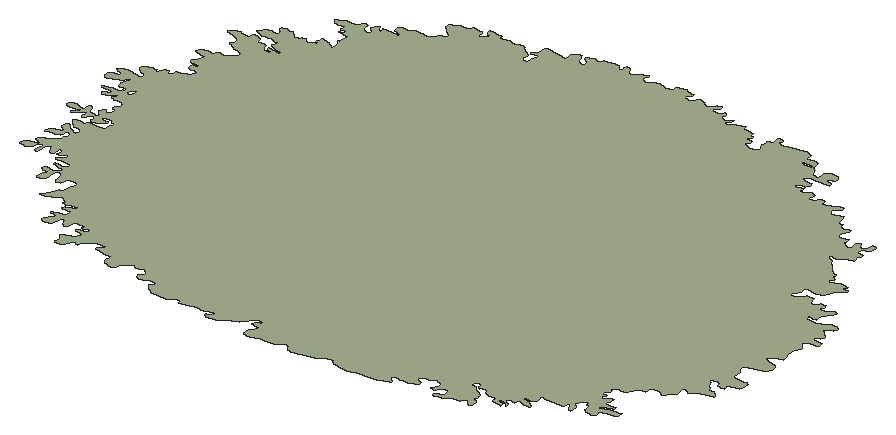
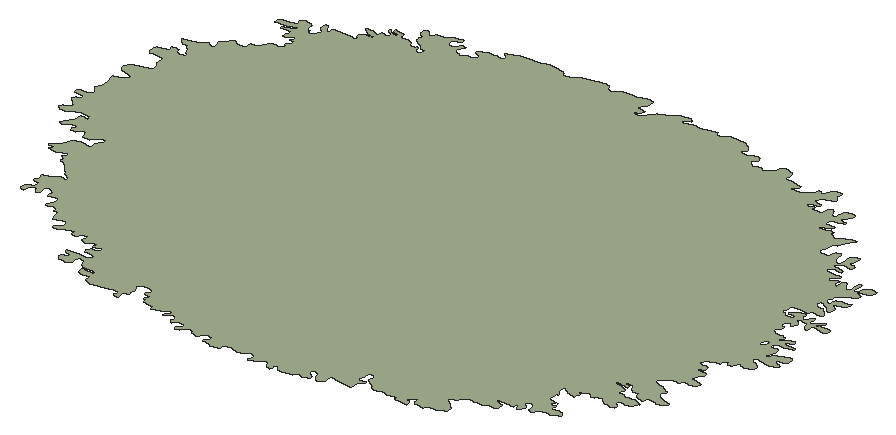
# SketchUp Ruby script. Lengths in inches.
U = 1.inch
M = Sketchup.active_model
def pt(a) = Geom::Point3d.new(a.map { |v| v * U })
def face(e, loops, mat)
  f = e.add_face(loops[0].map { |a| pt(a) })
  loops[1..].each { |l| e.add_face(l.map { |a| pt(a) }).erase! }
  f.material = f.back_material = mat if mat
  f
end
# faces: each face lists its corners as indices into pts; further lists are holes
def faces(e, pts, list, mat = nil) = list.each { |f| face(e, (f[0].is_a?(Array) ? f : [f]).map { |l| l.map { |i| pts[i] } }, mat) }
# xy, xz, yz: faces in a plane at the given z, y or x. An outline is a flat list of corners, or four numbers for a rectangle; further outlines are holes
def ring(l) = l.size == 4 ? [[l[0], l[1]], [l[2], l[1]], [l[2], l[3]], [l[0], l[3]]] : l.each_slice(2).to_a
def flat(e, list, mat, &to3) = list.each { |f| face(e, (f[0].is_a?(Array) ? f : [f]).map { |l| ring(l).map { |u, v| to3.(u, v) } }, mat) }
def xy(e, z, list, mat = nil) = flat(e, list, mat) { |x, y| [x, y, z] }
def xz(e, y, list, mat = nil) = flat(e, list, mat) { |x, z| [x, y, z] }
def yz(e, x, list, mat = nil) = flat(e, list, mat) { |y, z| [x, y, z] }
def lines(e, pts, list) = list.each { |a, b| e.add_line(pt(pts[a]), pt(pts[b])) }
# prism: a flat outline (further loops are holes) pulled along v
def prism(e, loops, v, mat = nil)
  f = face(e, loops, mat); d = Geom::Vector3d.new(v.map { |x| x * U })
  f.pushpull(f.normal.samedirection?(d) ? d.length : -d.length)
end
def box(e, o, s, mat = nil) = prism(e, [[o, [o[0] + s[0], o[1], o[2]], [o[0] + s[0], o[1] + s[1], o[2]], [o[0], o[1] + s[1], o[2]]]], [0, 0, s[2]], mat)
def at(x, y, z, deg = 0) = Geom::Transformation.translation(pt([x, y, z])) * Geom::Transformation.rotation(ORIGIN, Z_AXIS, deg.degrees)
def axes(o, x, y, z) = Geom::Transformation.new([*x, 0, *y, 0, *z, 0, *pt(o).to_a, 1])
def part(name) = M.definitions.add(name)
# library, detail: a bought-in or finely detailed component or shape, given as its bounding box
def library(name, o, s) = part(name).tap { |d| box(d.entities, o, s) }
def detail(e, o, s) = box(e.add_group.entities, o, s)
def put(e, d, t, mat = nil) = e.add_instance(d, t).tap { |i| i.material = mat if mat }
def group(e, t, mat = nil) = e.add_group.tap { |g| g.transformation = t; g.material = mat if mat }.entities
root = M.entities
M.materials.add("Boxwoodplan").color = [166, 177, 144]
xy(root,9.058,[[[199.667,67.129,199.556,67.133,199.461,67.159,199.405,67.215,199.403,67.317,199.429,67.382,199.493,67.445,199.542,67.509,199.6,67.606,199.414,67.635,199.324,67.644,199.344,67.732,199.43,67.79,199.461,67.8,199.456,67.846,199.367,67.877,199.251,67.837,199.154,67.706,199.011,67.551,198.85,67.464,198.745,67.441,198.684,67.416,198.668,67.373,198.524,67.281,198.33,67.251,198.241,67.26,198.161,67.306,198.161,67.328,198.206,67.359,198.297,67.437,198.365,67.483,198.276,67.498,198.163,67.48,198.043,67.436,197.947,67.445,197.85,67.454,197.753,67.447,197.626,67.403,197.426,67.356,197.337,67.349,197.299,67.443,197.291,67.465,197.224,67.473,197.135,67.454,196.966,67.336,196.766,67.328,196.536,67.353,196.369,67.446,196.228,67.61,196.411,67.702,196.311,67.756,196.175,67.772,196.049,67.749,195.977,67.697,195.896,67.672,195.78,67.738,195.738,67.806,195.826,67.847,195.852,67.907,195.857,67.957,195.816,68.009,195.744,68.085,195.658,68.117,195.571,68.064,195.505,68.038,195.449,68.08,195.432,68.103,195.408,68.121,195.379,68.111,195.299,68.058,195.228,68.01,195.152,67.923,195.14,67.79,195.069,67.749,195.019,67.723,194.959,67.725,194.86,67.746,194.773,67.793,194.729,67.861,194.721,67.951,194.73,68.018,194.743,68.04,194.724,68.08,194.51,68.1,194.578,68.135,194.552,68.136,194.459,68.13,194.289,68.146,194.212,68.173,194.195,68.206,194.21,68.224,194.335,68.314,194.333,68.371,194.248,68.393,194.089,68.39,193.958,68.319,193.861,68.233,193.786,68.199,193.739,68.172,193.738,68.154,193.774,68.101,193.758,68.046,193.688,68.081,193.624,68.121,193.563,68.072,193.541,68.017,193.509,67.904,193.462,67.855,193.389,67.822,193.298,67.816,193.228,67.841,193.209,67.874,193.216,67.892,193.237,67.932,193.259,67.991,193.228,68.048,193.127,68.149,193.241,68.229,193.302,68.269,193.382,68.285,193.449,68.315,193.504,68.37,193.589,68.476,193.517,68.503,193.4375,68.511,193.305,68.53,193.267,68.565,193.274,68.584,193.349,68.62,193.511,68.657,193.553,68.709,193.548,68.748,193.522,68.764,193.372,68.711,193.326,68.732,193.327,68.752,193.35,68.814,193.189,68.825,193.108,68.833,193.054,68.826,193.047,68.806,193.031,68.71,193.016,68.642,192.974,68.591,192.927,68.578,192.908,68.594,192.849,68.639,192.804,68.757,192.765,68.783,192.738,68.784,192.684,68.777,192.677,68.757,192.675,68.641,192.621,68.523,192.56,68.449,192.48,68.419,192.401,68.422,192.355,68.448,192.322,68.506,192.322,68.564,192.376,68.677,192.49,68.784,192.51,68.803,192.497,68.823,192.47,68.829,192.39,68.847,192.309,68.86,192.282,68.875,192.289,68.895,192.309,68.914,192.458,68.982,192.62,69.005,192.662,69.108,192.635,69.169,192.588,69.191,192.561,69.187,192.398,69.168,192.357,69.2,192.364,69.22,192.391,69.279,192.549,69.334,192.721,69.403,192.769,69.442,192.756,69.463,192.659,69.436,192.488,69.417,192.344,69.372,192.255,69.386,192.228,69.392,192.234,69.412,192.255,69.426,192.31,69.47,192.282,69.507,192.255,69.503,192.172,69.511,192.117,69.56,192.103,69.601,192.076,69.597,191.993,69.575,191.836,69.489,191.687,69.413,191.613,69.38,191.558,69.392,191.571,69.412,191.59,69.452,191.617,69.469,191.641,69.55,191.691,69.65,191.723,69.759,191.774,69.812,191.847,69.852,191.891,69.972,191.913,70.112,191.933,70.227,191.929,70.285,191.884,70.321,191.803,70.335,191.717,70.335,191.643,70.31,191.633,70.245,191.634,70.184,191.601,70.124,191.513,70.087,191.456,70.096,191.418,70.155,191.407,70.216,191.381,70.337,191.376,70.4,191.335,70.453,191.308,70.475,191.27,70.491,191.211,70.479,191.177,70.46,191.175,70.428,191.167,70.366,191.17,70.229,191.195,70.167,191.187,70.103,191.136,70.038,191.088,70.01,191.05,69.998,191.012,70.003,190.97,70.011,190.952,70.039,190.948,70.166,190.969,70.223,191.014,70.276,191.03,70.306,191.022,70.334,190.965,70.34,190.883,70.346,190.846,70.362,190.823,70.39,190.82,70.453,190.835,70.483,190.87,70.499,191.042,70.472,191.121,70.497,191.17,70.526,191.231,70.573,191.244,70.636,191.221,70.662,191.177,70.664,191.1,70.67,191.008,70.681,190.907,70.717,190.888,70.746,190.894,70.76,190.913,70.763,190.973,70.775,191.148,70.761,191.238,70.787,191.25,70.844,191.224,70.907,191.152,70.946,191.073,70.953,190.96,70.946,190.86,70.921,190.777,70.939,190.773,70.968,190.793,70.997,190.84,71.054,190.906,71.11,190.959,71.19,190.951,71.224,190.906,71.241,190.841,71.24,190.723,71.14,190.683,71.141,190.649,71.161,190.671,71.22,190.687,71.287,190.644,71.35,190.604,71.366,190.584,71.367,190.578,71.352,190.582,71.306,190.579,71.164,190.538,71.102,190.499,71.108,190.464,71.131,190.366,71.262,190.342,71.327,190.317,71.355,190.302,71.344,190.246,71.293,190.211,71.234,190.231,71.103,190.236,71.037,190.216,70.971,190.166,70.962,190.132,70.978,190.122,71.023,190.142,71.155,190.151,71.233,190.151,71.27,190.136,71.282,190.121,71.272,190.042,71.237,190.002,71.183,189.993,71.12,189.954,71.077,189.817,70.987,189.777,70.977,189.733,70.986,189.653,71.026,189.633,71.056,189.637,71.089,189.67,71.151,189.767,71.237,189.857,71.263,189.947,71.263,190.042,71.267,189.981,71.318,189.83,71.404,189.813,71.466,189.866,71.503,189.958,71.573,190.077,71.635,190.195,71.709,190.231,71.723,190.257,71.746,190.283,71.789,190.286,71.882,190.319,72.003,190.32,72.065,190.299,72.086,190.277,72.095,190.214,72.109,190.181,72.104,190.177,72.088,190.189,71.996,190.147,71.934,190.099,71.899,190.022,71.871,189.951,71.858,189.79,71.833,189.755,71.839,189.742,71.853,189.742,71.86,189.751,71.901,189.768,71.947,189.81,71.995,189.879,72.042,189.938,72.063,189.996,72.065,190.035,72.068,190.055,72.075,190.078,72.096,190.073,72.121,190.019,72.151,189.951,72.207,189.919,72.264,189.915,72.331,189.928,72.382,189.98,72.426,190.006,72.432,190.017,72.425,190.037,72.411,190.08,72.35,190.129,72.304,190.257,72.226,190.331,72.192,190.366,72.177,190.386,72.184,190.41,72.206,190.417,72.222,190.428,72.263,190.413,72.32,190.37,72.366,190.338,72.389,190.304,72.401,190.244,72.401,190.17,72.404,190.127,72.446,190.041,72.519,189.982,72.569,189.943,72.617,189.944,72.646,189.968,72.671,190.024,72.698,190.059,72.703,190.1,72.7,190.16,72.679,190.222,72.677,190.258,72.684,190.292,72.726,190.341,72.757,190.4,72.764,190.471,72.764,190.625,72.771,190.765,72.792,190.798,72.808,190.799,72.826,190.793,72.868,190.781,72.913,190.792,72.957,190.822,73.06,190.809,73.083,190.786,73.097,190.729,73.126,190.676,73.164,190.603,73.192,190.53,73.195,190.48,73.184,190.459,73.17,190.434,73.119,190.439,73.098,190.45,73.093,190.474,73.088,190.625,73.076,190.651,73.071,190.656,73.0625,190.647,73.046,190.607,73.007,190.562,72.964,190.497,72.928,190.435,72.884,190.363,72.849,190.326,72.852,190.306,72.863,190.281,72.9,190.274,72.995,190.257,73.02,190.275,73.034,190.281,73.077,190.275,73.088,190.264,73.088,190.249,73.087,190.223,73.083,190.191,73.076,190.173,73.065,190.092,72.97,190.06,72.915,190.029,72.892,190.006,72.895,189.98,72.916,189.971,72.932,189.965,72.973,189.994,73.057,189.999,73.102,189.99,73.13,189.97,73.137,189.932,73.128,189.912,73.114,189.866,73.064,189.744,72.957,189.708,72.932,189.682,72.927,189.645,72.935,189.633,72.951,189.724,73.057,189.787,73.102,189.801,73.129,189.8,73.145,189.791,73.152,189.78,73.148,189.765,73.143,189.734,73.131,189.65,73.108,189.483,73.089,189.41,73.096,189.362,73.121,189.34,73.149,189.339,73.165,189.356,73.217,189.404,73.264,189.464,73.281,189.535,73.284,189.609,73.266,189.737,73.223,189.823,73.197,189.834,73.201,189.834,73.22,189.825,73.239,189.8,73.287,189.799,73.342,189.806,73.407,189.818,73.437,189.835,73.45,189.884,73.413,189.923,73.363,189.95,73.317,189.96,73.255,189.972,73.204,189.987,73.176,190.01,73.175,190.145,73.157,190.218,73.144,190.253,73.14,190.271,73.154,190.286,73.202,190.231,73.244,190.172,73.309,190.155,73.335,190.155,73.352,190.189,73.46,190.219,73.483,190.246,73.489,190.261,73.477,190.27,73.459,190.299,73.414,190.31,73.39,190.322,73.391,190.343,73.404,190.423,73.482,190.44,73.528,190.441,73.579,190.427,73.611,190.406,73.623,190.343,73.646,190.303,73.666,190.295,73.687,190.311,73.736,190.367,73.773,190.401,73.795,190.414,73.816,190.422,73.869,190.42,73.916,190.325,73.992,190.181,74.014,190.119,74.031,190.084,74.013,190.056,74.014,189.987,74.031,189.968,74.058,189.977,74.082,190.103,74.185,190.097,74.217,190.075,74.233,190.03,74.225,190.001,74.216,189.875,74.154,189.835,74.107,189.786,74.063,189.717,74.049,189.689,74.05,189.642,74.102,189.67,74.126,189.6875,74.165,189.719,74.188,189.813,74.22,189.858,74.25,189.847,74.281,189.834,74.283,189.824,74.276,189.798,74.27,189.759,74.273,189.624,74.284,189.477,74.3125,189.453,74.327,189.459,74.347,189.484,74.375,189.697,74.435,189.76,74.434,189.821,74.419,189.881,74.391,189.908,74.393,189.914,74.403,189.963,74.48,189.987,74.495,189.993,74.515,189.993,74.583,189.982,74.593,189.969,74.591,189.911,74.591,189.854,74.585,189.807,74.568,189.783,74.576,189.762,74.596,189.737,74.63,189.717,74.718,189.728,74.806,189.758,74.848,189.764,74.88,189.777,74.923,189.814,74.944,189.81,74.99,189.788,75.026,189.699,75.003,189.681,74.969,189.682,74.95,189.685,74.886,189.605,74.839,189.464,74.745,189.308,74.7,189.224,74.725,189.182,74.778,189.173,74.904,189.301,74.99,189.384,75.003,189.427,75.027,189.451,75.061,189.45,75.081,189.364,75.112,189.291,75.138,189.229,75.194,189.264,75.249,189.34,75.278,189.436,75.312,189.501,75.311,189.68,75.267,189.772,75.246,189.857,75.25,189.908,75.269,189.914,75.289,189.898,75.355,189.837,75.407,189.792,75.415,189.68,75.485,189.633,75.527,189.619,75.564,189.612,75.617,189.612,75.644,189.625,75.659,189.667,75.695,189.718,75.709,189.832,75.741,189.863,75.751,189.903,75.75,189.953,75.746,189.966,75.733,189.981,75.703,189.995,75.689,190.005,75.689,190.033,75.692,190.049,75.704,190.07,75.754,190.098,75.787,190.114,75.81,190.117,75.835,190.133,75.86,190.153,75.872,190.201,75.884,190.24,75.877,190.261,75.833,190.265,75.781,190.282,75.755,190.303,75.754,190.345,75.796,190.37,75.838,190.384,75.942,190.4,75.968,190.432,75.975,190.464,75.974,190.483,75.963,190.504,75.94,190.536,75.94,190.589,75.961,190.633,76.007,190.647,76.032,190.636,76.046,190.696,76.043,190.725,76.046,190.741,76.066,190.746,76.114,190.78,76.155,190.814,76.2,190.76,76.243,190.693,76.272,190.656,76.271,190.623,76.261,190.581,76.249,190.539,76.255,190.517,76.271,190.496,76.295,190.473,76.397,190.486,76.423,190.491,76.439,190.501,76.443,190.606,76.463,190.652,76.472,190.67,76.483,190.66,76.486,190.574,76.514,190.508,76.526,190.48,76.519,190.445,76.52,190.409,76.52,190.373,76.532,190.335,76.582,190.317,76.611,190.317,76.642,190.332,76.663,190.361,76.678,190.392,76.697,190.4,76.725,190.43,76.782,190.457,76.836,190.463,76.89,190.456,76.917,190.416,76.928,190.338,76.954,190.165,77.001,190.129,77.018,190.112,77.042,190.148,77.097,190.192,77.131,190.238,77.159,190.293,77.178,190.345,77.1875,190.398,77.184,190.453,77.16,190.508,77.162,190.535,77.167,190.548,77.187,190.565,77.228,190.602,77.264,190.623,77.282,190.649,77.284,190.718,77.267,190.78,77.256,190.806,77.253,190.83,77.268,190.917,77.336,191.004,77.401,191.058,77.498,191.054,77.542,191.013,77.579,190.896,77.617,190.77,77.647,190.684,77.719,190.626,77.755,190.557,77.776,190.53,77.788,190.516,77.808,190.538,77.855,190.586,77.896,190.584,77.981,190.534,78.06,190.404,78.116,190.116,78.212,190.095,78.246,190.167,78.31,190.288,78.362,190.393,78.367,190.45,78.353,190.494,78.327,190.543,78.317,190.596,78.326,190.657,78.337,190.686,78.368,190.701,78.448,190.718,78.483,190.772,78.482,190.829,78.471,190.877,78.451,190.944,78.392,190.968,78.358,190.982,78.318,190.983,78.249,190.989,78.245,190.998,78.249,191.025,78.262,191.076,78.268,191.165,78.271,191.245,78.235,191.279,78.17,191.304,78.092,191.374,78.047,191.414,78.035,191.432,78.034,191.459,78.043,191.554,78.05,191.571,78.055,191.551,78.071,191.488,78.095,191.436,78.099,191.398,78.118,191.379,78.152,191.376,78.164,191.379,78.184,191.394,78.191,191.429,78.192,191.471,78.185,191.577,78.156,191.692,78.152,191.744,78.159,191.762,78.162,191.788,78.173,191.744,78.203,191.703,78.213,191.617,78.228,191.559,78.242,191.518,78.244,191.496,78.248,191.471,78.263,191.419,78.289,191.372,78.315,191.35,78.348,191.36,78.404,191.389,78.442,191.43,78.471,191.39,78.502,191.335,78.517,191.292,78.52,191.237,78.528,191.206,78.555,191.188,78.591,191.174,78.6,191.145,78.599,191.029,78.571,190.977,78.557,190.928,78.559,190.88,78.562,190.831,78.578,190.783,78.595,190.743,78.602,190.657,78.65,190.682,78.662,190.684,78.669,190.695,78.709,190.711,78.745,190.737,78.782,190.768,78.814,190.812,78.839,190.865,78.862,190.91,78.873,191.016,78.867,191.093,78.862,191.126,78.858,191.137,78.857,191.137,78.87,191.129,78.912,191.108,78.956,191.072,78.995,191.029,79.026,190.996,79.073,190.998,79.096,191.009,79.117,191.056,79.147,191.108,79.17,191.135,79.169,191.161,79.163,191.215,79.148,191.283,79.142,191.33,79.127,191.354,79.114,191.372,79.095,191.416,79.055,191.455,79.02,191.5,78.989,191.556,78.976,191.61,78.981,191.655,79.01,191.687,79.046,191.736,79.084,191.762,79.083,191.784,79.069,191.825,79.027,191.872,78.994,192,79.019,192.074,79.037,192.115,79.065,192.121,79.085,192.1,79.102,192.049,79.124,192.039,79.147,192.047,79.169,192.063,79.214,192.07,79.273,192.074,79.299,192.097,79.315,192.124,79.316,192.154,79.308,192.196,79.288,192.33,79.248,192.391,79.226,192.43,79.193,192.457,79.153,192.472,79.13,192.479,79.123,192.488,79.126,192.496,79.131,192.529,79.176,192.535,79.212,192.525,79.315,192.503,79.362,192.479,79.397,192.444,79.436,192.434,79.466,192.445,79.477,192.456,79.475,192.478,79.476,192.477,79.484,192.482,79.508,192.475,79.549,192.46,79.705,192.462,79.782,192.347,79.802,192.25,79.804,192.1875,79.8125,192.17,79.819,192.156,79.83,192.169,79.839,192.282,79.882,192.316,79.911,192.315,79.924,192.292,79.948,192.256,79.952,192.203,79.94,192.155,79.918,192.138,79.919,192.123,79.945,192.149,80.028,192.152,80.069,192.151,80.082,192.127,80.103,192.038,80.085,191.925,80.088,191.816,80.105,191.755,80.185,191.753,80.213,191.791,80.25,191.887,80.303,191.936,80.33,191.99,80.335,192.115,80.332,192.206,80.337,192.266,80.346,192.306,80.384,192.346,80.418,192.354,80.461,192.38,80.5,192.436,80.513,192.473,80.509,192.516,80.475,192.527,80.389,192.534,80.3,192.558,80.257,192.613,80.231,192.705,80.212,192.76,80.234,192.778,80.276,192.755,80.319,192.708,80.355,192.652,80.442,192.688,80.521,192.762,80.603,192.781,80.606,192.805,80.576,192.824,80.528,192.898,80.447,192.926,80.421,192.917,80.475,192.899,80.57,192.955,80.587,193.016,80.582,193.143,80.578,193.256,80.575,193.378,80.557,193.396,80.557,193.384,80.587,193.333,80.629,193.203,80.681,193.165,80.689,193.142,80.735,193.144,80.826,193.179,80.871,193.228,80.896,193.344,80.901,193.441,80.91,193.536,80.977,193.662,80.982,193.778,80.971,193.874,80.953,193.995,80.946,194.038,80.991,194.051,81.038,194.094,81.133,194.183,81.187,194.303,81.244,194.315,81.26,194.298,81.294,194.257,81.332,194.15,81.413,194.082,81.487,194.024,81.528,193.967,81.57,193.998,81.577,193.997,81.591,193.992,81.612,193.981,81.679,193.984,81.709,194.019,81.744,194.102,81.785,194.185,81.821,194.223,81.827,194.279,81.826,194.366,81.816,194.389,81.808,194.413,81.81,194.445,81.843,194.497,81.918,194.533,81.932,194.59,81.936,194.692,81.93,194.788,81.898,194.82,81.877,194.849,81.835,194.85,81.765,194.853,81.736,194.858,81.715,194.881,81.704,194.934,81.715,194.979,81.745,195.041,81.798,195.066,81.822,195.087,81.834,195.1,81.85,195.015,81.897,194.977,81.913,194.934,81.956,194.909,82.036,194.91,82.067,194.968,82.083,195.16,82.055,195.257,82.039,195.292,82.026,195.292,81.98,195.302,81.952,195.362,81.948,195.466,81.962,195.568,81.975,195.61,81.971,195.657,81.957,195.684,81.934,195.709,81.933,195.734,81.943,195.878,81.972,195.919,81.981,195.971,81.987,196.007,81.984,196.052,81.957,196.082,81.886,196.108,81.863,196.153,81.844,196.193,81.833,196.233,81.808,196.285,81.753,196.339,81.696,196.326,81.619,196.319,81.545,196.333,81.515,196.364,81.485,196.391,81.461,196.438,81.453,196.474,81.45,196.519,81.481,196.532,81.512,196.533,81.553,196.521,81.628,196.558,81.787,196.547,81.817,196.529,81.829,196.505,81.833,196.466,81.834,196.414,81.828,196.378,81.826,196.331,81.835,196.306,81.858,196.313,81.88,196.341,81.896,196.38,81.91,196.425,81.937,196.45,82.013,196.454,82.178,196.454,82.21,196.477,82.228,196.503,82.233,196.602,82.222,196.801,82.201,196.892,82.19,196.981,82.169,197.068,82.153,197.119,82.147,197.114,82.355,197.182,82.427,197.267,82.486,197.321,82.477,197.349,82.441,197.397,82.37,197.42,82.297,197.428,82.26,197.426,82.241,197.453,82.206,197.558,82.173,197.61,82.173,197.649,82.204,197.652,82.279,197.549,82.36,197.471,82.419,197.483,82.453,197.527,82.49,197.621,82.541,197.671,82.55,197.752,82.538,197.856,82.537,197.879,82.615,198.089,82.643,198.189,82.661,198.297,82.647,198.376,82.578,198.409,82.543,198.436,82.541,198.476,82.568,198.474,82.643,198.465,82.685,198.478,82.72,198.528,82.729,198.583,82.715,198.654,82.621,198.675,82.548,198.708,82.513,198.757,82.498,198.808,82.503,198.854,82.53,198.942,82.613,199.023,82.668,199.125,82.715,199.173,82.7,199.187,82.663,199.135,82.592,199.109,82.557,199.117,82.515,199.206,82.457,199.306,82.443,199.356,82.452,199.406,82.498,199.484,82.566,199.599,82.581,199.714,82.553,199.745,82.523,199.822,82.492,199.922,82.511,200.004,82.565,200.004,82.678,200.061,82.721,200.174,82.745,200.279,82.74,200.36,82.681,200.506,82.66,200.56,82.651,200.566,82.614,200.492,82.546,200.459,82.473,200.471,82.437,200.543,82.396,200.645,82.401,200.698,82.433,200.718,82.472,200.738,82.544,200.787,82.567,200.811,82.579,200.862,82.579,200.965,82.541,201.008,82.47,201.094,82.417,201.224,82.447,201.259,82.478,201.265,82.52,201.305,82.603,201.412,82.622,201.442,82.592,201.448,82.55,201.395,82.466,201.347,82.448,201.32,82.413,201.38,82.349,201.511,82.337,201.602,82.373,201.669,82.444,201.694,82.45,201.703,82.433,201.721,82.392,201.745,82.357,201.734,82.301,201.714,82.257,201.732,82.222,201.821,82.179,201.929,82.184,201.984,82.203,202.035,82.258,202.052,82.273,202.054,82.255,202.041,82.212,201.968,82.132,201.934,82.102,201.945,82.066,201.992,82.047,202.05,82.048,202.146,82.088,202.228,82.146,202.448,82.225,202.47,82.153,202.493,82.123,202.544,82.118,202.66,82.11,202.784,82.084,202.799,82.013,202.822,81.983,202.868,81.964,202.891,81.93,202.877,81.892,202.85,81.795,202.967,81.773,203.013,81.755,203.023,81.72,202.949,81.65,202.935,81.613,202.951,81.579,203.027,81.527,203.13,81.5,203.231,81.496,203.343,81.563,203.385,81.639,203.327,81.71,203.294,81.779,203.314,81.885,203.323,81.922,203.294,81.956,203.29,81.992,203.332,82.018,203.433,82.022,203.422,82.122,203.38,82.274,203.43,82.287,203.495,82.275,203.548,82.256,203.579,82.199,203.529,82.131,203.533,82.095,203.579,82.076,203.687,82.076,203.817,82.111,204.324,82.178,204.37,82.168,204.416,82.145,204.462,82.121,204.496,82.097,204.527,82.027,204.51,81.935,204.714,81.949,204.779,81.943,204.864,81.911,204.901,81.805,204.886,81.757,204.87,81.724,204.829,81.717,204.659,81.749,204.595,81.755,204.552,81.755,204.532,81.749,204.529,81.733,204.557,81.685,204.598,81.666,204.645,81.666,204.818,81.681,204.887,81.683,204.971,81.648,205.008,81.609,205.039,81.546,205.107,81.437,205.186,81.398,205.271,81.394,205.302,81.435,205.296,81.518,205.278,81.571,205.285,81.637,205.326,81.687,205.427,81.719,205.536,81.732,205.625,81.701,205.673,81.659,205.707,81.597,205.708,81.551,205.646,81.495,205.58,81.482,205.539,81.471,205.507,81.437,205.511,81.407,205.56,81.389,205.658,81.363,205.729,81.339,205.749,81.306,205.737,81.275,205.683,81.247,205.596,81.24,205.434,81.233,205.347,81.222,205.258,81.256,205.194,81.269,205.112,81.251,205.056,81.208,205.054,81.143,205.112,81.103,205.199,81.081,205.285,81.066,205.332,81.066,205.366,81.046,205.387,81.003,205.37,80.938,205.335,80.89,205.307,80.866,205.262,80.854,205.12,80.834,205.1,80.829,205.091,80.784,205.095,80.751,205.14,80.732,205.207,80.731,205.248,80.731,205.298,80.746,205.361,80.778,205.375,80.712,205.346,80.665,205.339,80.635,205.378,80.617,205.439,80.622,205.521,80.67,205.577,80.711,205.605,80.736,205.643,80.721,205.707,80.704,205.776,80.651,205.772,80.603,205.729,80.537,205.696,80.472,205.714,80.448,205.761,80.445,205.837,80.456,205.919,80.495,205.958,80.554,206.03,80.597,206.09,80.609,206.127,80.601,206.145,80.577,206.148,80.548,206.131,80.521,206.103,80.497,206.105,80.483,206.126,80.481,206.298,80.499,206.379,80.51,206.446,80.552,206.488,80.589,206.567,80.614,206.664,80.619,206.687,80.595,206.69,80.566,206.53,80.349,206.545,80.304,206.602,80.251,206.685,80.237,206.774,80.255,206.842,80.283,206.927,80.305,206.992,80.213,207.028,79.999,207.03,79.985,207.066,79.974,207.15,79.996,207.161,79.918,207.185,79.871,207.261,79.861,207.398,79.896,207.466,79.893,207.481,79.839,207.413,79.619,207.402,79.567,207.425,79.514,207.491,79.486,207.559,79.496,207.695,79.523,207.715,79.419,207.71,79.316,207.832,79.247,207.965,79.216,207.995,79.318,207.985,79.421,207.962,79.474,207.99,79.525,208.059,79.535,208.098,79.482,208.12,79.429,208.168,79.395,208.245,79.418,208.299,79.467,208.323,79.583,208.327,79.636,208.388,79.659,208.445,79.631,208.475,79.577,208.45,79.455,208.335,79.375,208.282,79.339,208.261,79.282,208.241,79.231,208.264,79.186,208.396,79.161,208.452,79.134,208.457,79.083,208.384,78.997,208.419,78.895,208.448,78.844,208.436,78.794,208.302,78.768,208.201,78.729,208.097,78.658,208.046,78.623,207.98,78.626,207.916,78.659,207.884,78.667,207.858,78.643,207.902,78.549,208.021,78.483,208.068,78.445,208.065,78.396,208.15,78.32,208.316,78.132,208.448,78.05,208.511,78.035,208.548,77.992,208.533,77.898,208.649,77.834,208.586,77.749,208.566,77.697,208.564,77.673,208.595,77.661,208.732,77.679,208.867,77.755,208.997,77.768,209.122,77.734,209.125,77.687,209.059,77.66,209.033,77.644,209.047,77.62,209.125,77.599,209.197,77.596,209.229,77.595,209.242,77.571,209.154,77.482,208.988,77.322,208.964,77.232,208.96,77.187,208.932,77.142,208.839,77.067,208.711,77.038,208.586,77.043,208.477,77.082,208.408,77.076,208.381,77.004,208.408,76.894,208.379,76.787,208.261,76.72,208.289,76.62,208.427,76.642,208.599,76.833,208.826,76.815,208.902,76.605,208.947,76.595,209.029,76.618,209.116,76.723,209.254,76.735,209.292,76.635,209.242,76.574,209.227,76.539,209.304,76.501,209.443,76.531,209.5625,76.598,209.609,76.614,209.699,76.592,209.677,76.477,209.566,76.384,209.501,76.289,209.509,76.113,209.495,76.078,209.402,76.056,209.27,76.087,209.295,75.981,209.426,75.941,209.572,75.936,209.721,75.965,209.958,76.087,210.094,76.099,210.186,76.008,210.153,75.905,210.013,75.849,209.966,75.825,209.9375,75.766,210.041,75.675,210.192,75.515,210.159,75.414,210.043,75.359,210.007,75.335,210.045,75.274,210.189,75.269,210.319,75.247,210.331,75.145,210.258,75.089,210.125,75.078,210,75.041,209.957,74.942,210.125,74.761,210.018,74.568,210.021,74.388,210.075,74.176,210.119,74.078,209.987,74.051,209.864,74.008,209.77,73.931,209.743,73.869,209.854,73.801,210.106,73.744,210.183,73.662,210.204,73.559,210.162,73.467,210.047,73.394,209.586,73.234,209.588,73.141,209.632,73.048,209.686,72.954,209.6875,72.863,209.682,72.803,209.679,72.773,209.705,72.719,209.826,72.676,209.951,72.672,210.077,72.682,210.119,72.68,210.177,72.633,210.188,72.453,210.161,72.395,210.052,72.347,209.925,72.33,209.884,72.331,209.838,72.281,209.88,72.191,209.867,72.163,209.782,72.144,209.741,72.145,209.671,72.17,209.639,72.26,209.569,72.292,209.446,72.297,209.404,72.291,209.388,72.233,209.464,72.156,209.551,71.992,209.579,71.969,209.605,71.918,209.623,71.888,209.704,71.877,209.784,71.86,209.869,71.792,209.932,71.71,209.929,71.681,209.845,71.656,209.596,71.616,209.401,71.488,209.328,71.469,209.233,71.544,209.193,71.553,209.129,71.52,209.132,71.435,209.188,71.27,209.146,71.264,209.113,71.219,209.064,71.18,209.01,71.066,208.971,71.019,208.937,71,208.901,71.013,208.779,71.1,208.716,71.115,208.673,71.116,208.628,71.098,208.565,71.063,208.535,70.991,208.545,70.938,208.527,70.874,208.365,70.852,208.313,70.81,208.281,70.759,208.234,70.718,208.222,70.655,208.191,70.609,208.157,70.583,208.12,70.573,208.051,70.564,207.953,70.575,207.893,70.55,207.831,70.502,207.801,70.457,207.876,70.419,207.903,70.376,207.867,70.32,207.812,70.284,207.791,70.225,207.79,70.209,207.789,70.194,207.808,70.186,207.88,70.18,207.906,70.182,207.926,70.182,207.93,70.166,207.892,70.097,207.873,70.049,207.87,70.02,207.911,70.018,208.05,70.094,208.119,70.11,208.2,70.107,208.184,70.004,208.166,69.89,208.166,69.843,208.189,69.82,208.229,69.818,208.293,69.845,208.374,69.846,208.433,69.832,208.473,69.827,208.479,69.798,208.439,69.76,208.36,69.73,208.294,69.722,208.211,69.696,208.172,69.658,208.155,69.602,208.159,69.587,208.199,69.586,208.281,69.611,208.439,69.673,208.593,69.703,208.719,69.705,208.771,69.685,208.746,69.611,208.725,69.569,208.664,69.518,208.511,69.492,208.372,69.491,208.311,69.482,208.28,69.427,208.306,69.308,208.291,69.264,208.21,69.243,208.074,69.255,208.016,69.261,207.972,69.314,207.963,69.426,207.963,69.468,207.951,69.496,207.942,69.511,207.922,69.512,207.864,69.525,207.859,69.581,207.861,69.595,207.857,69.61,207.838,69.614,207.758,69.617,207.701,69.591,207.656,69.536,207.619,69.499,207.594,69.44,207.605,69.391,207.661,69.354,207.736,69.254,207.732,69.155,207.723,69.115,207.716,69.088,207.685,69.066,207.665,69.067,207.644,69.098,207.615,69.157,207.55,69.258,207.509,69.298,207.495,69.312,207.484,69.299,207.477,69.271,207.474,69.227,207.455,69.173,207.449,69.16,207.419,69.144,207.336,69.137,207.195,69.139,206.909,69.14,206.851,69.162,206.764,69.173,206.745,69.163,206.739,69.133,206.789,69.074,206.814,68.976,206.808,68.936,206.776,68.896,206.752,68.889,206.692,68.88,206.589,68.88,206.491,68.884,206.443,68.853,206.498,68.829,206.599,68.814,206.707,68.78,206.782,68.726,206.863,68.654,206.845,68.629,206.784,68.614,206.683,68.621,206.646,68.63,206.595,68.65,206.547,68.684,206.497,68.708,206.462,68.63,206.452,68.558,206.412,68.545,206.356,68.558,206.311,68.589,206.298,68.6,206.28,68.608,206.268,68.59,206.234,68.513,206.236,68.485,206.269,68.448,206.361,68.416,206.4,68.383,206.413,68.34,206.411,68.326,206.392,68.323,206.349,68.36,206.269,68.409,206.176,68.427,206.119,68.429,206.107,68.415,206.128,68.39,206.242,68.347,206.279,68.335,206.302,68.292,206.298,68.264,206.297,68.251,206.254,68.249,206.141,68.26,206.036,68.295,206.001,68.325,205.992,68.371,205.991,68.441,205.94,68.461,205.881,68.442,205.781,68.449,205.682,68.467,205.655,68.489,205.63,68.526,205.634,68.568,205.64,68.583,205.602,68.591,205.508,68.616,205.451,68.619,205.416,68.606,205.404,68.577,205.384,68.571,205.357,68.597,205.354,68.612,205.384,68.635,205.4,68.646,205.392,68.671,205.305,68.729,205.268,68.752,205.249,68.756,205.208,68.736,205.168,68.716,205.148,68.71,205.137,68.681,205.16,68.59,205.255,68.587,205.294,68.582,205.324,68.541,205.317,68.513,205.311,68.499,205.319,68.471,205.43,68.434,205.518,68.396,205.579,68.338,205.596,68.3125,205.595,68.299,205.56,68.283,205.54,68.273,205.571,68.251,205.626,68.225,205.638,68.2,205.587,68.168,205.575,68.141,205.6,68.106,205.685,68.062,205.763,67.994,205.762,67.851,205.741,67.825,205.689,67.814,205.635,67.829,205.597,67.874,205.557,67.939,205.539,67.949,205.501,67.944,205.449,67.926,205.427,67.897,205.428,67.854,205.427,67.84,205.394,67.828,205.217,67.819,205.209,67.826,205.161,67.808,205.117,67.777,205.033,67.692,204.981,67.661,204.907,67.651,204.769,67.643,204.715,67.658,204.713,67.698,204.822,67.762,204.922,67.834,204.919,67.937,204.913,67.98,204.913,67.994,204.882,68.015,204.822,68.034,204.748,68.034,204.664,67.95,204.644,67.911,204.587,67.866,204.572,67.857,204.536,67.865,204.499,67.88,204.487,67.907,204.527,67.999,204.587,68.094,204.588,68.135,204.52,68.189,204.409,68.224,204.357,68.246,204.32,68.238,204.295,68.215,204.261,68.171,204.228,68.156,204.186,68.157,204.13,68.166,204.093,68.168,204.055,68.145,203.974,68.05,203.988,68.01,204.062,67.97,204.117,67.938,204.144,67.917,204.153,67.89,204.129,67.851,204.069,67.807,203.967,67.756,203.912,67.735,203.839,67.738,203.784,67.76,203.71,67.769,203.665,67.745,203.628,67.743,203.596,67.76,203.541,67.766,203.468,67.752,203.446,67.717,203.456,67.659,203.553,67.575,203.58,67.536,203.581,67.51,203.581,67.497,203.563,67.492,203.273,67.391,202.998,67.369,202.765,67.373,202.674,67.371,202.552,67.31,202.449,67.275,202.352,67.279,202.314,67.281,202.265,67.299,202.217,67.328,202.156,67.325,202.067,67.334,201.983,67.376,201.923,67.433,201.892,67.478,201.833,67.491,201.734,67.479,201.638,67.438,201.558,67.398,201.459,67.325,201.362,67.269,201.269,67.24,201.028,67.222,200.838,67.186,200.741,67.19,200.676,67.284,200.645,67.351,200.557,67.365,200.466,67.352,200.37,67.28,200.305,67.217,200.215,67.21,200.038,67.233,199.853,67.24,199.775,67.189],[190.175,74.415,190.217,74.419,190.237,74.422,190.263,74.431,190.275,74.474,190.276,74.513,190.283,74.597,190.275,74.631,190.263,74.643,190.263,74.658,190.22,74.635,190.164,74.612,190.144,74.606,190.128,74.59,190.107,74.557,190.097,74.52,190.099,74.476,190.118,74.437,190.137,74.421]]],"Boxwoodplan")
